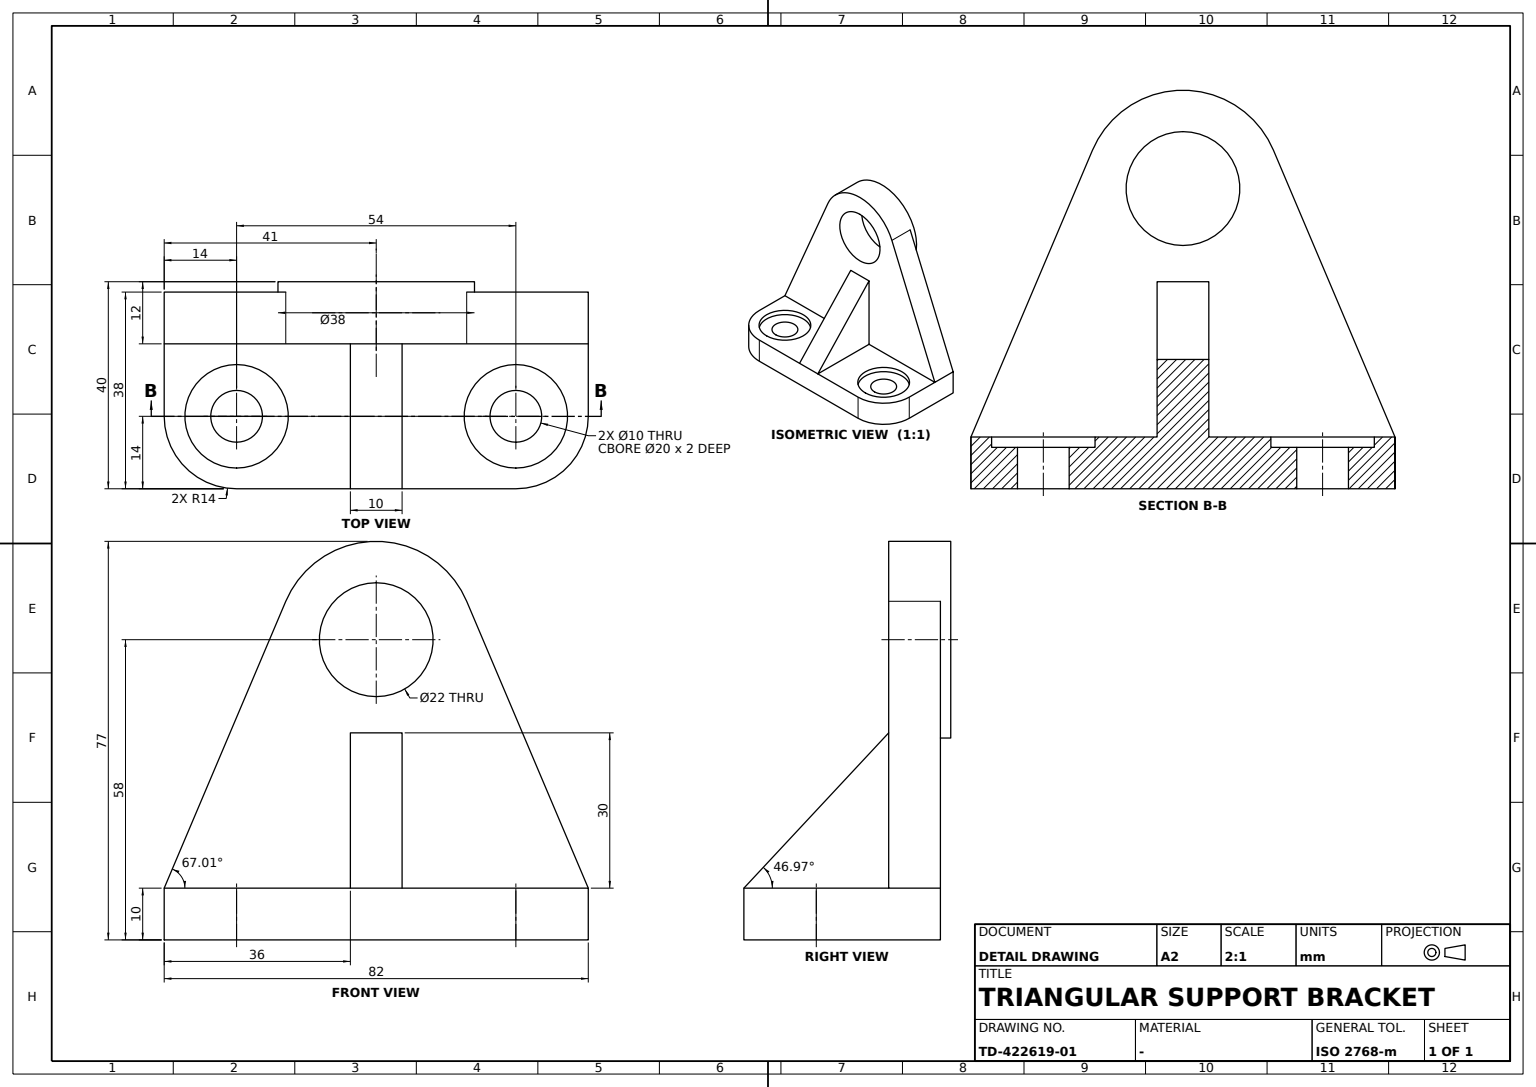
ISO-10303-21;
HEADER;
FILE_DESCRIPTION((''),'2;1');
FILE_NAME('','',(''),(''),'','','');
FILE_SCHEMA(('AUTOMOTIVE_DESIGN'));
ENDSEC;
DATA;
#1=APPLICATION_CONTEXT('');
#2=PRODUCT_CONTEXT('',#1,'mechanical');
#3=PRODUCT('','','',(#2));
#4=PRODUCT_DEFINITION_FORMATION('','',#3);
#5=PRODUCT_DEFINITION_CONTEXT('',#1,'design');
#6=PRODUCT_DEFINITION('','',#4,#5);
#7=PRODUCT_DEFINITION_SHAPE('','',#6);
#8=(LENGTH_UNIT()NAMED_UNIT(*)SI_UNIT(.MILLI.,.METRE.));
#9=(NAMED_UNIT(*)PLANE_ANGLE_UNIT()SI_UNIT($,.RADIAN.));
#10=(NAMED_UNIT(*)SI_UNIT($,.STERADIAN.)SOLID_ANGLE_UNIT());
#11=UNCERTAINTY_MEASURE_WITH_UNIT(LENGTH_MEASURE(0.005),#8,'distance_accuracy_value','');
#12=(GEOMETRIC_REPRESENTATION_CONTEXT(3)GLOBAL_UNCERTAINTY_ASSIGNED_CONTEXT((#11))GLOBAL_UNIT_ASSIGNED_CONTEXT((#8,#9,#10))REPRESENTATION_CONTEXT('',''));
#13=CARTESIAN_POINT('',(-9.,5.,5.));
#14=VERTEX_POINT('',#13);
#15=CARTESIAN_POINT('',(19.,5.,5.));
#16=VERTEX_POINT('',#15);
#17=CARTESIAN_POINT('',(0.,5.,5.));
#18=DIRECTION('',(1.,0.,0.));
#19=VECTOR('',#18,1000.);
#20=LINE('',#17,#19);
#21=EDGE_CURVE('',#14,#16,#20,.T.);
#22=ORIENTED_EDGE('',*,*,#21,.F.);
#23=CARTESIAN_POINT('',(-9.,5.,35.));
#24=VERTEX_POINT('',#23);
#25=CARTESIAN_POINT('',(-9.,5.,0.));
#26=DIRECTION('',(0.,0.,-1.));
#27=VECTOR('',#26,1000.);
#28=LINE('',#25,#27);
#29=EDGE_CURVE('',#24,#14,#28,.T.);
#30=ORIENTED_EDGE('',*,*,#29,.F.);
#31=DIRECTION('',(-0.68231825,0.,0.731055268));
#32=VECTOR('',#31,1000.);
#33=LINE('',#15,#32);
#34=EDGE_CURVE('',#16,#24,#33,.T.);
#35=ORIENTED_EDGE('',*,*,#34,.F.);
#36=EDGE_LOOP('',(#22,#30,#35));
#37=FACE_BOUND('',#36,.T.);
#38=CARTESIAN_POINT('',(0.,5.,0.));
#39=DIRECTION('',(0.,1.,0.));
#40=DIRECTION('',(-1.,0.,0.));
#41=AXIS2_PLACEMENT_3D('',#38,#39,#40);
#42=PLANE('',#41);
#43=ADVANCED_FACE('',(#37),#42,.T.);
#44=CARTESIAN_POINT('',(19.,27.,-5.));
#45=VERTEX_POINT('',#44);
#46=CARTESIAN_POINT('',(5.,41.,-5.));
#47=VERTEX_POINT('',#46);
#48=CARTESIAN_POINT('',(5.,27.,-5.));
#49=DIRECTION('',(0.,0.,1.));
#50=AXIS2_PLACEMENT_3D('',#48,#49,#18);
#51=CIRCLE('',#50,14.);
#52=EDGE_CURVE('',#45,#47,#51,.T.);
#53=ORIENTED_EDGE('',*,*,#52,.T.);
#54=CARTESIAN_POINT('',(5.,41.,5.));
#55=VERTEX_POINT('',#54);
#56=CARTESIAN_POINT('',(5.,41.,0.));
#57=VECTOR('',#49,1000.);
#58=LINE('',#56,#57);
#59=EDGE_CURVE('',#47,#55,#58,.T.);
#60=ORIENTED_EDGE('',*,*,#59,.T.);
#61=CARTESIAN_POINT('',(19.,27.,5.));
#62=VERTEX_POINT('',#61);
#63=CARTESIAN_POINT('',(5.,27.,5.));
#64=AXIS2_PLACEMENT_3D('',#63,#49,#18);
#65=CIRCLE('',#64,14.);
#66=EDGE_CURVE('',#62,#55,#65,.T.);
#67=ORIENTED_EDGE('',*,*,#66,.F.);
#68=CARTESIAN_POINT('',(19.,27.,0.));
#69=LINE('',#68,#57);
#70=EDGE_CURVE('',#45,#62,#69,.T.);
#71=ORIENTED_EDGE('',*,*,#70,.F.);
#72=EDGE_LOOP('',(#53,#60,#67,#71));
#73=FACE_BOUND('',#72,.T.);
#74=CARTESIAN_POINT('',(5.,27.,0.));
#75=AXIS2_PLACEMENT_3D('',#74,#49,#39);
#76=CYLINDRICAL_SURFACE('',#75,14.);
#77=ADVANCED_FACE('',(#73),#76,.T.);
#78=CARTESIAN_POINT('',(19.,-5.,5.));
#79=VERTEX_POINT('',#78);
#80=CARTESIAN_POINT('',(-9.,-5.,35.));
#81=VERTEX_POINT('',#80);
#82=LINE('',#78,#32);
#83=EDGE_CURVE('',#79,#81,#82,.T.);
#84=ORIENTED_EDGE('',*,*,#83,.F.);
#85=CARTESIAN_POINT('',(19.,41.,5.));
#86=VECTOR('',#39,1000.);
#87=LINE('',#85,#86);
#88=EDGE_CURVE('',#79,#16,#87,.T.);
#89=ORIENTED_EDGE('',*,*,#88,.T.);
#90=ORIENTED_EDGE('',*,*,#34,.T.);
#91=CARTESIAN_POINT('',(-9.,0.,35.));
#92=LINE('',#91,#86);
#93=EDGE_CURVE('',#81,#24,#92,.T.);
#94=ORIENTED_EDGE('',*,*,#93,.F.);
#95=EDGE_LOOP('',(#84,#89,#90,#94));
#96=FACE_BOUND('',#95,.T.);
#97=CARTESIAN_POINT('',(19.,0.,5.));
#98=DIRECTION('',(0.731055268,0.,0.68231825));
#99=DIRECTION('',(0.68231825,0.,-0.731055268));
#100=AXIS2_PLACEMENT_3D('',#97,#98,#99);
#101=PLANE('',#100);
#102=ADVANCED_FACE('',(#96),#101,.T.);
#103=CARTESIAN_POINT('',(-19.,41.,5.));
#104=VERTEX_POINT('',#103);
#105=CARTESIAN_POINT('',(-9.,41.,5.));
#106=VERTEX_POINT('',#105);
#107=LINE('',#103,#19);
#108=EDGE_CURVE('',#104,#106,#107,.T.);
#109=ORIENTED_EDGE('',*,*,#108,.F.);
#110=CARTESIAN_POINT('',(-19.,17.491367,60.419709));
#111=VERTEX_POINT('',#110);
#112=CARTESIAN_POINT('',(-19.,30.292613,30.241802));
#113=DIRECTION('',(0.,-0.390511011,0.920598257));
#114=VECTOR('',#113,1000.);
#115=LINE('',#112,#114);
#116=EDGE_CURVE('',#104,#111,#115,.T.);
#117=ORIENTED_EDGE('',*,*,#116,.T.);
#118=CARTESIAN_POINT('',(-9.,17.491367,60.419709));
#119=VERTEX_POINT('',#118);
#120=CARTESIAN_POINT('',(-15.,17.491367,60.419709));
#121=LINE('',#120,#19);
#122=EDGE_CURVE('',#119,#111,#121,.F.);
#123=ORIENTED_EDGE('',*,*,#122,.F.);
#124=LINE('',#105,#114);
#125=EDGE_CURVE('',#106,#119,#124,.T.);
#126=ORIENTED_EDGE('',*,*,#125,.F.);
#127=EDGE_LOOP('',(#109,#117,#123,#126));
#128=FACE_BOUND('',#127,.T.);
#129=DIRECTION('',(0.,0.920598257,0.390511011));
#130=AXIS2_PLACEMENT_3D('',#103,#129,#113);
#131=PLANE('',#130);
#132=ADVANCED_FACE('',(#128),#131,.T.);
#133=CARTESIAN_POINT('',(-9.,0.,64.));
#134=VERTEX_POINT('',#133);
#135=CARTESIAN_POINT('',(-9.,0.,53.));
#136=AXIS2_PLACEMENT_3D('',#135,#40,#49);
#137=CIRCLE('',#136,11.);
#138=EDGE_CURVE('',#134,#134,#137,.F.);
#139=ORIENTED_EDGE('',*,*,#138,.F.);
#140=EDGE_LOOP('',(#139));
#141=FACE_BOUND('',#140,.T.);
#142=CARTESIAN_POINT('',(-9.,-5.,5.));
#143=VERTEX_POINT('',#142);
#144=CARTESIAN_POINT('',(-9.,-5.,0.));
#145=LINE('',#144,#27);
#146=EDGE_CURVE('',#81,#143,#145,.T.);
#147=ORIENTED_EDGE('',*,*,#146,.F.);
#148=ORIENTED_EDGE('',*,*,#93,.T.);
#149=ORIENTED_EDGE('',*,*,#29,.T.);
#150=CARTESIAN_POINT('',(-9.,0.,5.));
#151=LINE('',#150,#86);
#152=EDGE_CURVE('',#14,#106,#151,.T.);
#153=ORIENTED_EDGE('',*,*,#152,.T.);
#154=ORIENTED_EDGE('',*,*,#125,.T.);
#155=CARTESIAN_POINT('',(-9.,-17.491367,60.419709));
#156=VERTEX_POINT('',#155);
#157=CIRCLE('',#136,19.);
#158=EDGE_CURVE('',#119,#156,#157,.F.);
#159=ORIENTED_EDGE('',*,*,#158,.T.);
#160=CARTESIAN_POINT('',(-9.,-41.,5.));
#161=VERTEX_POINT('',#160);
#162=DIRECTION('',(0.,-0.390511011,-0.920598257));
#163=VECTOR('',#162,1000.);
#164=LINE('',#160,#163);
#165=EDGE_CURVE('',#156,#161,#164,.T.);
#166=ORIENTED_EDGE('',*,*,#165,.T.);
#167=EDGE_CURVE('',#161,#143,#151,.T.);
#168=ORIENTED_EDGE('',*,*,#167,.T.);
#169=EDGE_LOOP('',(#147,#148,#149,#153,#154,#159,#166,#168));
#170=FACE_BOUND('',#169,.T.);
#171=CARTESIAN_POINT('',(-9.,0.,0.));
#172=DIRECTION('',(0.,-1.,0.));
#173=AXIS2_PLACEMENT_3D('',#171,#40,#172);
#174=PLANE('',#173);
#175=ADVANCED_FACE('',(#141,#170),#174,.F.);
#176=ORIENTED_EDGE('',*,*,#122,.T.);
#177=CARTESIAN_POINT('',(-19.,-17.491367,60.419709));
#178=VERTEX_POINT('',#177);
#179=CARTESIAN_POINT('',(-19.,0.,53.));
#180=AXIS2_PLACEMENT_3D('',#179,#18,#26);
#181=CIRCLE('',#180,19.);
#182=EDGE_CURVE('',#111,#178,#181,.F.);
#183=ORIENTED_EDGE('',*,*,#182,.T.);
#184=CARTESIAN_POINT('',(-15.,-17.491367,60.419709));
#185=LINE('',#184,#19);
#186=EDGE_CURVE('',#156,#178,#185,.F.);
#187=ORIENTED_EDGE('',*,*,#186,.F.);
#188=ORIENTED_EDGE('',*,*,#158,.F.);
#189=EDGE_LOOP('',(#176,#183,#187,#188));
#190=FACE_BOUND('',#189,.T.);
#191=CARTESIAN_POINT('',(-21.,0.,34.));
#192=VERTEX_POINT('',#191);
#193=CARTESIAN_POINT('',(-21.,0.,53.));
#194=AXIS2_PLACEMENT_3D('',#193,#18,#26);
#195=CIRCLE('',#194,19.);
#196=EDGE_CURVE('',#192,#192,#195,.T.);
#197=ORIENTED_EDGE('',*,*,#196,.T.);
#198=EDGE_LOOP('',(#197));
#199=FACE_BOUND('',#198,.T.);
#200=CARTESIAN_POINT('',(-15.,0.,53.));
#201=AXIS2_PLACEMENT_3D('',#200,#18,#39);
#202=CYLINDRICAL_SURFACE('',#201,19.);
#203=ADVANCED_FACE('',(#190,#199),#202,.T.);
#204=ORIENTED_EDGE('',*,*,#165,.F.);
#205=ORIENTED_EDGE('',*,*,#186,.T.);
#206=CARTESIAN_POINT('',(-19.,-41.,5.));
#207=VERTEX_POINT('',#206);
#208=CARTESIAN_POINT('',(-19.,-42.797519,0.762494));
#209=LINE('',#208,#163);
#210=EDGE_CURVE('',#178,#207,#209,.T.);
#211=ORIENTED_EDGE('',*,*,#210,.T.);
#212=VECTOR('',#40,1000.);
#213=LINE('',#206,#212);
#214=EDGE_CURVE('',#161,#207,#213,.T.);
#215=ORIENTED_EDGE('',*,*,#214,.F.);
#216=EDGE_LOOP('',(#204,#205,#211,#215));
#217=FACE_BOUND('',#216,.T.);
#218=DIRECTION('',(0.,-0.920598257,0.390511011));
#219=AXIS2_PLACEMENT_3D('',#206,#218,#162);
#220=PLANE('',#219);
#221=ADVANCED_FACE('',(#217),#220,.T.);
#222=CARTESIAN_POINT('',(15.,-27.,3.));
#223=VERTEX_POINT('',#222);
#224=CARTESIAN_POINT('',(5.,-27.,3.));
#225=AXIS2_PLACEMENT_3D('',#224,#49,#18);
#226=CIRCLE('',#225,10.);
#227=EDGE_CURVE('',#223,#223,#226,.T.);
#228=ORIENTED_EDGE('',*,*,#227,.F.);
#229=EDGE_LOOP('',(#228));
#230=FACE_BOUND('',#229,.T.);
#231=CARTESIAN_POINT('',(15.,-27.,5.));
#232=VERTEX_POINT('',#231);
#233=CARTESIAN_POINT('',(5.,-27.,5.));
#234=AXIS2_PLACEMENT_3D('',#233,#49,#18);
#235=CIRCLE('',#234,10.);
#236=EDGE_CURVE('',#232,#232,#235,.T.);
#237=ORIENTED_EDGE('',*,*,#236,.T.);
#238=EDGE_LOOP('',(#237));
#239=FACE_BOUND('',#238,.T.);
#240=CARTESIAN_POINT('',(5.,-27.,4.));
#241=AXIS2_PLACEMENT_3D('',#240,#49,#39);
#242=CYLINDRICAL_SURFACE('',#241,10.);
#243=ADVANCED_FACE('',(#230,#239),#242,.F.);
#244=ORIENTED_EDGE('',*,*,#227,.T.);
#245=EDGE_LOOP('',(#244));
#246=FACE_BOUND('',#245,.T.);
#247=CARTESIAN_POINT('',(10.,-27.,3.));
#248=VERTEX_POINT('',#247);
#249=CIRCLE('',#225,5.);
#250=EDGE_CURVE('',#248,#248,#249,.T.);
#251=ORIENTED_EDGE('',*,*,#250,.F.);
#252=EDGE_LOOP('',(#251));
#253=FACE_BOUND('',#252,.T.);
#254=CARTESIAN_POINT('',(0.,0.,3.));
#255=AXIS2_PLACEMENT_3D('',#254,#49,#39);
#256=PLANE('',#255);
#257=ADVANCED_FACE('',(#246,#253),#256,.T.);
#258=CARTESIAN_POINT('',(10.,27.,3.));
#259=VERTEX_POINT('',#258);
#260=CARTESIAN_POINT('',(5.,27.,3.));
#261=AXIS2_PLACEMENT_3D('',#260,#49,#18);
#262=CIRCLE('',#261,5.);
#263=EDGE_CURVE('',#259,#259,#262,.T.);
#264=ORIENTED_EDGE('',*,*,#263,.T.);
#265=EDGE_LOOP('',(#264));
#266=FACE_BOUND('',#265,.T.);
#267=CARTESIAN_POINT('',(10.,27.,-5.));
#268=VERTEX_POINT('',#267);
#269=CIRCLE('',#50,5.);
#270=EDGE_CURVE('',#268,#268,#269,.T.);
#271=ORIENTED_EDGE('',*,*,#270,.F.);
#272=EDGE_LOOP('',(#271));
#273=FACE_BOUND('',#272,.T.);
#274=CARTESIAN_POINT('',(5.,27.,-1.66));
#275=AXIS2_PLACEMENT_3D('',#274,#49,#39);
#276=CYLINDRICAL_SURFACE('',#275,5.);
#277=ADVANCED_FACE('',(#266,#273),#276,.F.);
#278=CARTESIAN_POINT('',(15.,27.,3.));
#279=VERTEX_POINT('',#278);
#280=CIRCLE('',#261,10.);
#281=EDGE_CURVE('',#279,#279,#280,.T.);
#282=ORIENTED_EDGE('',*,*,#281,.T.);
#283=EDGE_LOOP('',(#282));
#284=FACE_BOUND('',#283,.T.);
#285=ORIENTED_EDGE('',*,*,#263,.F.);
#286=EDGE_LOOP('',(#285));
#287=FACE_BOUND('',#286,.T.);
#288=ADVANCED_FACE('',(#284,#287),#256,.T.);
#289=CARTESIAN_POINT('',(15.,27.,5.));
#290=VERTEX_POINT('',#289);
#291=CIRCLE('',#64,10.);
#292=EDGE_CURVE('',#290,#290,#291,.T.);
#293=ORIENTED_EDGE('',*,*,#292,.F.);
#294=EDGE_LOOP('',(#293));
#295=FACE_BOUND('',#294,.T.);
#296=ORIENTED_EDGE('',*,*,#152,.F.);
#297=ORIENTED_EDGE('',*,*,#21,.T.);
#298=VECTOR('',#172,1000.);
#299=LINE('',#97,#298);
#300=EDGE_CURVE('',#62,#16,#299,.T.);
#301=ORIENTED_EDGE('',*,*,#300,.F.);
#302=ORIENTED_EDGE('',*,*,#66,.T.);
#303=CARTESIAN_POINT('',(0.,41.,5.));
#304=LINE('',#303,#19);
#305=EDGE_CURVE('',#106,#55,#304,.T.);
#306=ORIENTED_EDGE('',*,*,#305,.F.);
#307=EDGE_LOOP('',(#296,#297,#301,#302,#306));
#308=FACE_BOUND('',#307,.T.);
#309=CARTESIAN_POINT('',(0.,0.,5.));
#310=AXIS2_PLACEMENT_3D('',#309,#49,#39);
#311=PLANE('',#310);
#312=ADVANCED_FACE('',(#295,#308),#311,.T.);
#313=CARTESIAN_POINT('',(19.,-27.,-5.));
#314=VERTEX_POINT('',#313);
#315=CARTESIAN_POINT('',(19.,0.,-5.));
#316=LINE('',#315,#298);
#317=EDGE_CURVE('',#45,#314,#316,.T.);
#318=ORIENTED_EDGE('',*,*,#317,.F.);
#319=ORIENTED_EDGE('',*,*,#70,.T.);
#320=ORIENTED_EDGE('',*,*,#300,.T.);
#321=ORIENTED_EDGE('',*,*,#88,.F.);
#322=CARTESIAN_POINT('',(19.,-27.,5.));
#323=VERTEX_POINT('',#322);
#324=EDGE_CURVE('',#79,#323,#299,.T.);
#325=ORIENTED_EDGE('',*,*,#324,.T.);
#326=CARTESIAN_POINT('',(19.,-27.,0.));
#327=LINE('',#326,#57);
#328=EDGE_CURVE('',#314,#323,#327,.T.);
#329=ORIENTED_EDGE('',*,*,#328,.F.);
#330=EDGE_LOOP('',(#318,#319,#320,#321,#325,#329));
#331=FACE_BOUND('',#330,.T.);
#332=CARTESIAN_POINT('',(19.,41.,0.));
#333=AXIS2_PLACEMENT_3D('',#332,#40,#172);
#334=PLANE('',#333);
#335=ADVANCED_FACE('',(#331),#334,.F.);
#336=CARTESIAN_POINT('',(5.,-41.,-5.));
#337=VERTEX_POINT('',#336);
#338=CARTESIAN_POINT('',(5.,-41.,5.));
#339=VERTEX_POINT('',#338);
#340=CARTESIAN_POINT('',(5.,-41.,0.));
#341=LINE('',#340,#57);
#342=EDGE_CURVE('',#337,#339,#341,.T.);
#343=ORIENTED_EDGE('',*,*,#342,.T.);
#344=CARTESIAN_POINT('',(0.,-41.,5.));
#345=LINE('',#344,#212);
#346=EDGE_CURVE('',#339,#161,#345,.T.);
#347=ORIENTED_EDGE('',*,*,#346,.T.);
#348=ORIENTED_EDGE('',*,*,#214,.T.);
#349=CARTESIAN_POINT('',(-19.,-41.,-5.));
#350=VERTEX_POINT('',#349);
#351=CARTESIAN_POINT('',(-19.,-41.,0.));
#352=LINE('',#351,#57);
#353=EDGE_CURVE('',#350,#207,#352,.T.);
#354=ORIENTED_EDGE('',*,*,#353,.F.);
#355=CARTESIAN_POINT('',(0.,-41.,-5.));
#356=LINE('',#355,#212);
#357=EDGE_CURVE('',#337,#350,#356,.T.);
#358=ORIENTED_EDGE('',*,*,#357,.F.);
#359=EDGE_LOOP('',(#343,#347,#348,#354,#358));
#360=FACE_BOUND('',#359,.T.);
#361=CARTESIAN_POINT('',(19.,-41.,0.));
#362=AXIS2_PLACEMENT_3D('',#361,#39,#40);
#363=PLANE('',#362);
#364=ADVANCED_FACE('',(#360),#363,.F.);
#365=ORIENTED_EDGE('',*,*,#292,.T.);
#366=EDGE_LOOP('',(#365));
#367=FACE_BOUND('',#366,.T.);
#368=ORIENTED_EDGE('',*,*,#281,.F.);
#369=EDGE_LOOP('',(#368));
#370=FACE_BOUND('',#369,.T.);
#371=CARTESIAN_POINT('',(5.,27.,4.));
#372=AXIS2_PLACEMENT_3D('',#371,#49,#39);
#373=CYLINDRICAL_SURFACE('',#372,10.);
#374=ADVANCED_FACE('',(#367,#370),#373,.F.);
#375=ORIENTED_EDGE('',*,*,#146,.T.);
#376=CARTESIAN_POINT('',(0.,-5.,5.));
#377=LINE('',#376,#19);
#378=EDGE_CURVE('',#143,#79,#377,.T.);
#379=ORIENTED_EDGE('',*,*,#378,.T.);
#380=ORIENTED_EDGE('',*,*,#83,.T.);
#381=EDGE_LOOP('',(#375,#379,#380));
#382=FACE_BOUND('',#381,.T.);
#383=CARTESIAN_POINT('',(0.,-5.,0.));
#384=AXIS2_PLACEMENT_3D('',#383,#39,#40);
#385=PLANE('',#384);
#386=ADVANCED_FACE('',(#382),#385,.F.);
#387=ORIENTED_EDGE('',*,*,#210,.F.);
#388=ORIENTED_EDGE('',*,*,#182,.F.);
#389=ORIENTED_EDGE('',*,*,#116,.F.);
#390=CARTESIAN_POINT('',(-19.,41.,-5.));
#391=VERTEX_POINT('',#390);
#392=CARTESIAN_POINT('',(-19.,41.,0.));
#393=LINE('',#392,#57);
#394=EDGE_CURVE('',#391,#104,#393,.T.);
#395=ORIENTED_EDGE('',*,*,#394,.F.);
#396=CARTESIAN_POINT('',(-19.,0.,-5.));
#397=LINE('',#396,#86);
#398=EDGE_CURVE('',#350,#391,#397,.T.);
#399=ORIENTED_EDGE('',*,*,#398,.F.);
#400=ORIENTED_EDGE('',*,*,#353,.T.);
#401=EDGE_LOOP('',(#387,#388,#389,#395,#399,#400));
#402=FACE_BOUND('',#401,.T.);
#403=AXIS2_PLACEMENT_3D('',#351,#18,#39);
#404=PLANE('',#403);
#405=ADVANCED_FACE('',(#402),#404,.F.);
#406=ORIENTED_EDGE('',*,*,#236,.F.);
#407=EDGE_LOOP('',(#406));
#408=FACE_BOUND('',#407,.T.);
#409=ORIENTED_EDGE('',*,*,#378,.F.);
#410=ORIENTED_EDGE('',*,*,#167,.F.);
#411=ORIENTED_EDGE('',*,*,#346,.F.);
#412=CIRCLE('',#234,14.);
#413=EDGE_CURVE('',#339,#323,#412,.T.);
#414=ORIENTED_EDGE('',*,*,#413,.T.);
#415=ORIENTED_EDGE('',*,*,#324,.F.);
#416=EDGE_LOOP('',(#409,#410,#411,#414,#415));
#417=FACE_BOUND('',#416,.T.);
#418=ADVANCED_FACE('',(#408,#417),#311,.T.);
#419=ORIENTED_EDGE('',*,*,#342,.F.);
#420=CARTESIAN_POINT('',(5.,-27.,-5.));
#421=AXIS2_PLACEMENT_3D('',#420,#49,#18);
#422=CIRCLE('',#421,14.);
#423=EDGE_CURVE('',#337,#314,#422,.T.);
#424=ORIENTED_EDGE('',*,*,#423,.T.);
#425=ORIENTED_EDGE('',*,*,#328,.T.);
#426=ORIENTED_EDGE('',*,*,#413,.F.);
#427=EDGE_LOOP('',(#419,#424,#425,#426));
#428=FACE_BOUND('',#427,.T.);
#429=CARTESIAN_POINT('',(5.,-27.,0.));
#430=AXIS2_PLACEMENT_3D('',#429,#49,#18);
#431=CYLINDRICAL_SURFACE('',#430,14.);
#432=ADVANCED_FACE('',(#428),#431,.T.);
#433=ORIENTED_EDGE('',*,*,#138,.T.);
#434=EDGE_LOOP('',(#433));
#435=FACE_BOUND('',#434,.T.);
#436=CARTESIAN_POINT('',(-21.,0.,42.));
#437=VERTEX_POINT('',#436);
#438=CIRCLE('',#194,11.);
#439=EDGE_CURVE('',#437,#437,#438,.T.);
#440=ORIENTED_EDGE('',*,*,#439,.F.);
#441=EDGE_LOOP('',(#440));
#442=FACE_BOUND('',#441,.T.);
#443=CYLINDRICAL_SURFACE('',#201,11.);
#444=ADVANCED_FACE('',(#435,#442),#443,.F.);
#445=CARTESIAN_POINT('',(10.,-27.,-5.));
#446=VERTEX_POINT('',#445);
#447=CIRCLE('',#421,5.);
#448=EDGE_CURVE('',#446,#446,#447,.T.);
#449=ORIENTED_EDGE('',*,*,#448,.F.);
#450=EDGE_LOOP('',(#449));
#451=FACE_BOUND('',#450,.T.);
#452=ORIENTED_EDGE('',*,*,#250,.T.);
#453=EDGE_LOOP('',(#452));
#454=FACE_BOUND('',#453,.T.);
#455=CARTESIAN_POINT('',(5.,-27.,-1.66));
#456=AXIS2_PLACEMENT_3D('',#455,#49,#39);
#457=CYLINDRICAL_SURFACE('',#456,5.);
#458=ADVANCED_FACE('',(#451,#454),#457,.F.);
#459=ORIENTED_EDGE('',*,*,#439,.T.);
#460=EDGE_LOOP('',(#459));
#461=FACE_BOUND('',#460,.T.);
#462=ORIENTED_EDGE('',*,*,#196,.F.);
#463=EDGE_LOOP('',(#462));
#464=FACE_BOUND('',#463,.T.);
#465=CARTESIAN_POINT('',(-21.,0.,0.));
#466=AXIS2_PLACEMENT_3D('',#465,#18,#39);
#467=PLANE('',#466);
#468=ADVANCED_FACE('',(#461,#464),#467,.F.);
#469=ORIENTED_EDGE('',*,*,#305,.T.);
#470=ORIENTED_EDGE('',*,*,#59,.F.);
#471=CARTESIAN_POINT('',(0.,41.,-5.));
#472=LINE('',#471,#19);
#473=EDGE_CURVE('',#391,#47,#472,.T.);
#474=ORIENTED_EDGE('',*,*,#473,.F.);
#475=ORIENTED_EDGE('',*,*,#394,.T.);
#476=ORIENTED_EDGE('',*,*,#108,.T.);
#477=EDGE_LOOP('',(#469,#470,#474,#475,#476));
#478=FACE_BOUND('',#477,.T.);
#479=AXIS2_PLACEMENT_3D('',#392,#172,#18);
#480=PLANE('',#479);
#481=ADVANCED_FACE('',(#478),#480,.F.);
#482=ORIENTED_EDGE('',*,*,#448,.T.);
#483=EDGE_LOOP('',(#482));
#484=FACE_BOUND('',#483,.T.);
#485=ORIENTED_EDGE('',*,*,#52,.F.);
#486=ORIENTED_EDGE('',*,*,#317,.T.);
#487=ORIENTED_EDGE('',*,*,#423,.F.);
#488=ORIENTED_EDGE('',*,*,#357,.T.);
#489=ORIENTED_EDGE('',*,*,#398,.T.);
#490=ORIENTED_EDGE('',*,*,#473,.T.);
#491=EDGE_LOOP('',(#485,#486,#487,#488,#489,#490));
#492=FACE_BOUND('',#491,.T.);
#493=ORIENTED_EDGE('',*,*,#270,.T.);
#494=EDGE_LOOP('',(#493));
#495=FACE_BOUND('',#494,.T.);
#496=CARTESIAN_POINT('',(0.,0.,-5.));
#497=AXIS2_PLACEMENT_3D('',#496,#49,#39);
#498=PLANE('',#497);
#499=ADVANCED_FACE('',(#484,#492,#495),#498,.F.);
#500=CLOSED_SHELL('',(#43,#77,#102,#132,#175,#203,#221,#243,#257,#277,#288,#312,#335,#364,#374,#386,#405,#418,#432,#444,#458,#468,#481,#499));
#501=MANIFOLD_SOLID_BREP('',#500);
#502=ADVANCED_BREP_SHAPE_REPRESENTATION('',(#501),#12);
#503=SHAPE_DEFINITION_REPRESENTATION(#7,#502);
ENDSEC;
END-ISO-10303-21;
